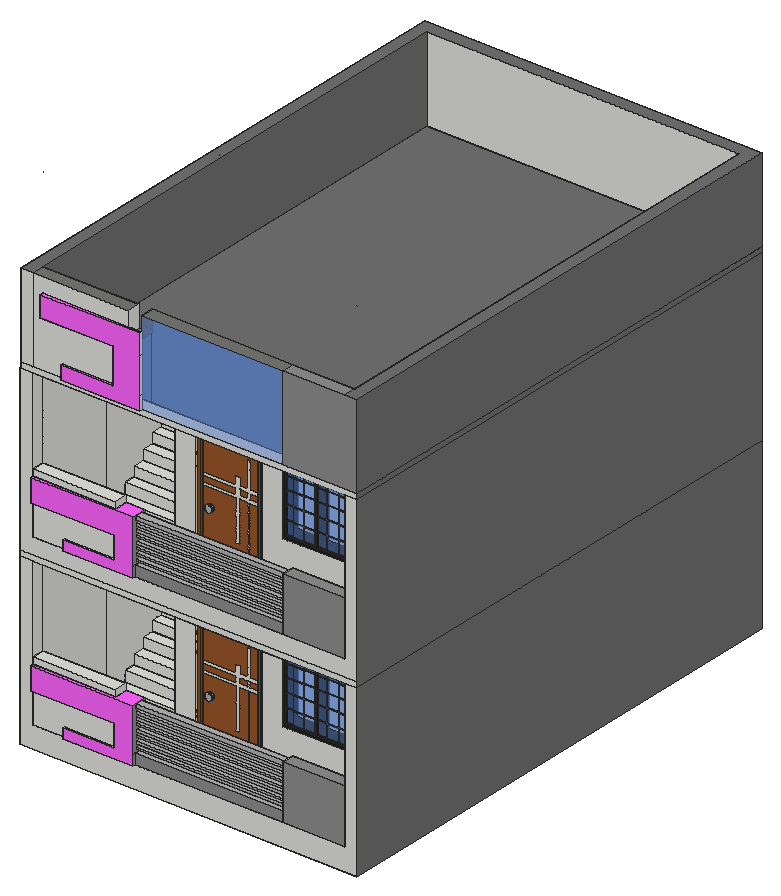
# SketchUp Ruby script. Lengths in inches.
U = 1.inch
M = Sketchup.active_model
def pt(a) = Geom::Point3d.new(a.map { |v| v * U })
def face(e, loops, mat)
  f = e.add_face(loops[0].map { |a| pt(a) })
  loops[1..].each { |l| e.add_face(l.map { |a| pt(a) }).erase! }
  f.material = f.back_material = mat if mat
  f
end
# faces: each face lists its corners as indices into pts; further lists are holes
def faces(e, pts, list, mat = nil) = list.each { |f| face(e, (f[0].is_a?(Array) ? f : [f]).map { |l| l.map { |i| pts[i] } }, mat) }
# xy, xz, yz: faces in a plane at the given z, y or x. An outline is a flat list of corners, or four numbers for a rectangle; further outlines are holes
def ring(l) = l.size == 4 ? [[l[0], l[1]], [l[2], l[1]], [l[2], l[3]], [l[0], l[3]]] : l.each_slice(2).to_a
def flat(e, list, mat, &to3) = list.each { |f| face(e, (f[0].is_a?(Array) ? f : [f]).map { |l| ring(l).map { |u, v| to3.(u, v) } }, mat) }
def xy(e, z, list, mat = nil) = flat(e, list, mat) { |x, y| [x, y, z] }
def xz(e, y, list, mat = nil) = flat(e, list, mat) { |x, z| [x, y, z] }
def yz(e, x, list, mat = nil) = flat(e, list, mat) { |y, z| [x, y, z] }
def lines(e, pts, list) = list.each { |a, b| e.add_line(pt(pts[a]), pt(pts[b])) }
# prism: a flat outline (further loops are holes) pulled along v
def prism(e, loops, v, mat = nil)
  f = face(e, loops, mat); d = Geom::Vector3d.new(v.map { |x| x * U })
  f.pushpull(f.normal.samedirection?(d) ? d.length : -d.length)
end
def box(e, o, s, mat = nil) = prism(e, [[o, [o[0] + s[0], o[1], o[2]], [o[0] + s[0], o[1] + s[1], o[2]], [o[0], o[1] + s[1], o[2]]]], [0, 0, s[2]], mat)
def at(x, y, z, deg = 0) = Geom::Transformation.translation(pt([x, y, z])) * Geom::Transformation.rotation(ORIGIN, Z_AXIS, deg.degrees)
def axes(o, x, y, z) = Geom::Transformation.new([*x, 0, *y, 0, *z, 0, *pt(o).to_a, 1])
def part(name) = M.definitions.add(name)
# library, detail: a bought-in or finely detailed component or shape, given as its bounding box
def library(name, o, s) = part(name).tap { |d| box(d.entities, o, s) }
def detail(e, o, s) = box(e.add_group.entities, o, s)
def put(e, d, t, mat = nil) = e.add_instance(d, t).tap { |i| i.material = mat if mat }
def group(e, t, mat = nil) = e.add_group.tap { |g| g.transformation = t; g.material = mat if mat }.entities
root = M.entities
M.materials.add("[Aluminum]").color = [179, 179, 179]
M.materials.add("[Color C07]").color = [153, 76, 0]
M.materials.add("[Color K03]").color = [255, 101, 255]
M.materials.add("[Color M04]").color = [142, 142, 142]
M.materials.add("[Color M05]").color = [114, 114, 114]
M.materials.add("[Color M08]").color = [30, 30, 30]
M.materials.add("[Metal Seamed]").color = [118, 119, 115]
M.materials.add("[Translucent Glass Blue]").color = [100, 149, 237]
M.materials["[Translucent Glass Blue]"].alpha = 0.5
M.materials.add("[Wood Cherry Original]").color = [152, 86, 42]
c1 = part("Group\#1")
xy(c1.entities,0,[[0,0,48,2],[0,2,48,11]],"[Color C07]")
xy(c1.entities,3,[[3,2,45,11]])
xy(c1.entities,3,[[3,0,45,2]],"[Color C07]")
xy(c1.entities,81,[[3,2,45,11]])
xy(c1.entities,81,[[3,0,45,2]],"[Color C07]")
xy(c1.entities,84,[[0,0,48,2],[0,2,48,11]],"[Color C07]")
xz(c1.entities,0,[[8.6,33.24,9.28,33.33,9.92,33.6,10.46,34.01,10.88,34.56,11.14,35.1875,11.23,35.87,11.14,36.55,10.88,37.18,10.46,37.72,9.92,38.14,9.28,38.4,8.6,38.49,7.92,38.4,7.29,38.14,6.75,37.72,6.33,37.18,6.07,36.55,5.98,35.87,6.07,35.1875,6.33,34.56,6.75,34.01,7.29,33.6,7.92,33.33]],"[Aluminum]")
xz(c1.entities,0,[[[0,0,48,84],[3,3,45,81]]],"[Color C07]")
xz(c1.entities,2,[[[0,0,48,84],[3,3,45,81]],[[35.64,15.58,37.45,15.58,37.45,48.41,45,48.41,45,50.73,37.45,50.73,37.45,54.78,45,54.78,45,57.1,37.45,57.1,37.45,75.83,35.64,75.83,35.64,57.1,29.69,57.1,29.69,62.31,27.44,62.31,27.44,57.1,3,57.1,3,54.78,27.44,54.78,27.44,50.73,3,50.73,3,48.41,27.44,48.41,27.44,19.68,29.69,19.68,29.69,48.41,35.64,48.41],[29.69,50.73,35.64,54.78]]])
xz(c1.entities,2,[[[3,3,45,3,45,48.41,37.45,48.41,37.45,15.58,35.64,15.58,35.64,48.41,29.69,48.41,29.69,19.68,27.44,19.68,27.44,48.41,3,48.41],[8.6,33.24,7.92,33.33,7.29,33.6,6.75,34.01,6.33,34.56,6.07,35.1875,5.98,35.87,6.07,36.55,6.33,37.18,6.75,37.72,7.29,38.14,7.92,38.4,8.6,38.49,9.28,38.4,9.92,38.14,10.46,37.72,10.88,37.18,11.14,36.55,11.23,35.87,11.14,35.1875,10.88,34.56,10.46,34.01,9.92,33.6,9.28,33.33]],[8.6,33.24,7.92,33.33,7.29,33.6,6.75,34.01,6.33,34.56,6.07,35.1875,5.98,35.87,6.07,36.55,6.33,37.18,6.75,37.72,7.29,38.14,7.92,38.4,8.6,38.49,9.28,38.4,9.92,38.14,10.46,37.72,10.88,37.18,11.14,36.55,11.23,35.87,11.14,35.1875,10.88,34.56,10.46,34.01,9.92,33.6,9.28,33.33],[3,50.73,27.44,54.78],[29.69,50.73,35.64,54.78],[37.45,50.73,45,54.78],
  [3,57.1,27.44,57.1,27.44,62.31,29.69,62.31,29.69,57.1,35.64,57.1,35.64,75.83,37.45,75.83,37.45,57.1,45,57.1,45,81,3,81]],"[Wood Cherry Original]")
xz(c1.entities,11,[[[0,0,48,84],[3,3,45,81]]])
yz(c1.entities,0,[[0,0,2,84],[2,0,11,84]],"[Color C07]")
yz(c1.entities,3,[[2,3,11,81]])
yz(c1.entities,3,[[0,3,2,81]],"[Color C07]")
yz(c1.entities,45,[[2,3,11,81]])
yz(c1.entities,45,[[0,3,2,81]],"[Color C07]")
yz(c1.entities,48,[[0,0,2,84],[2,0,11,84]],"[Color C07]")
p = [[7.92,2,33.33],[8.6,2,33.24],[8.6,0,33.24],[7.92,0,33.33],[9.28,2,33.33],[9.28,0,33.33],
  [7.29,2,33.6],[7.29,0,33.6],[9.92,2,33.6],[9.92,0,33.6],[6.75,2,34.01],[6.75,0,34.01],
  [10.46,2,34.01],[10.46,0,34.01],[6.33,2,34.56],[6.33,0,34.56],[10.88,2,34.56],[10.88,0,34.56],
  [6.07,2,35.1875],[6.07,0,35.1875],[11.14,2,35.1875],[11.14,0,35.1875],[5.98,2,35.87],[5.98,0,35.87],
  [11.23,2,35.87],[11.23,0,35.87],[6.07,2,36.55],[6.07,0,36.55],[11.14,2,36.55],[11.14,0,36.55],
  [6.33,2,37.18],[6.33,0,37.18],[10.88,2,37.18],[10.88,0,37.18],[6.75,2,37.72],[6.75,0,37.72],
  [10.46,2,37.72],[10.46,0,37.72],[7.29,2,38.14],[7.29,0,38.14],[9.92,2,38.14],[9.92,0,38.14],
  [7.92,2,38.4],[7.92,0,38.4],[9.28,2,38.4],[9.28,0,38.4],[8.6,2,38.49],[8.6,0,38.49]]
faces(c1.entities,p,[[0,1,2,3],[1,4,5,2],[6,0,3,7],[4,8,9,5],[10,6,7,11],[8,12,13,9],[14,10,11,15],[12,16,17,13],
  [18,14,15,19],[16,20,21,17],[22,18,19,23],[20,24,25,21],[26,22,23,27],[24,28,29,25],[30,26,27,31],[28,32,33,29],
  [34,30,31,35],[32,36,37,33],[38,34,35,39],[36,40,41,37],[42,38,39,43],[40,44,45,41],[46,42,43,47],[44,46,47,45]],"[Aluminum]")
c2 = part("Group\#2")
xy(c2.entities,0,[[0,0,48,11]])
xy(c2.entities,2,[[2,0,5.91,2],[5.91,0,6.35,2],[6.35,0,13.47,2],[13.47,0,13.91,2],[13.91,0,23.03,2],
  [24.15,0,29.6,2],[29.6,0,30.03,2],[30.03,0,38.16,2],[38.16,0,38.6,2],[38.6,0,46,2],
  [2,2,5.91,11],[5.91,2,6.35,11],[6.35,2,13.47,11],[13.47,2,13.91,11],[13.91,2,23.03,11],
  [24.15,2,29.6,11],[29.6,2,30.03,11],[30.03,2,38.16,11],[38.16,2,38.6,11],[38.6,2,46,11]])
xy(c2.entities,46,[[2,0,5.91,2],[5.91,0,6.35,2],[6.35,0,13.47,2],[13.47,0,13.91,2],[13.91,0,23.03,2],
  [24.15,0,29.6,2],[29.6,0,30.03,2],[30.03,0,38.16,2],[38.16,0,38.6,2],[38.6,0,46,2],
  [2,2,5.91,11],[5.91,2,6.35,11],[6.35,2,13.47,11],[13.47,2,13.91,11],[13.91,2,23.03,11],
  [24.15,2,29.6,11],[29.6,2,30.03,11],[30.03,2,38.16,11],[38.16,2,38.6,11],[38.6,2,46,11]])
xy(c2.entities,48,[[0,0,48,11]])
xz(c2.entities,0,[[[0,0,48,48],[24.15,2,46,46],[2,2,23.03,46]]],"[Color M08]")
xz(c2.entities,2,[[2,2,5.91,10.99],[[5.91,2,6.35,2,6.35,10.99,13.47,10.99,13.47,2,13.91,2,13.91,10.99,23.03,10.99,23.03,11.58,13.91,11.58,13.91,21.05,23.03,21.05,23.03,21.64,13.91,21.64,13.91,30.55,23.03,30.55,23.03,31.14,13.91,31.14,13.91,39.49,23.03,39.49,23.03,40.08,13.91,40.08,13.91,46,13.47,46,13.47,40.08,6.35,40.08,6.35,46,5.91,46,5.91,40.08,2,40.08,2,39.49,5.91,39.49,5.91,31.14,2,31.14,2,30.55,5.91,30.55,5.91,21.64,2,21.64,2,21.05,5.91,21.05,5.91,11.58,2,11.58,2,10.99,5.91,10.99],[6.35,11.58,13.47,21.05],[6.35,21.64,13.47,30.55],[6.35,31.14,13.47,39.49]],[6.35,2,13.47,10.99],[13.91,2,23.03,10.99],[24.15,2,29.6,10.99],
  [[29.6,2,30.03,2,30.03,10.99,38.16,10.99,38.16,2,38.6,2,38.6,10.99,46,10.99,46,11.58,38.6,11.58,38.6,21.05,46,21.05,46,21.64,38.6,21.64,38.6,30.55,46,30.55,46,31.14,38.6,31.14,38.6,39.49,46,39.49,46,40.08,38.6,40.08,38.6,46,38.16,46,38.16,40.08,30.03,40.08,30.03,46,29.6,46,29.6,40.08,24.15,40.08,24.15,39.49,29.6,39.49,29.6,31.14,24.15,31.14,24.15,30.55,29.6,30.55,29.6,21.64,24.15,21.64,24.15,21.05,29.6,21.05,29.6,11.58,24.15,11.58,24.15,10.99,29.6,10.99],[30.03,11.58,38.16,21.05],[30.03,21.64,38.16,30.55],[30.03,31.14,38.16,39.49]],[30.03,2,38.16,10.99],[38.6,2,46,10.99],[2,11.58,5.91,21.05],[6.35,11.58,13.47,21.05],
  [13.91,11.58,23.03,21.05],[24.15,11.58,29.6,21.05],[30.03,11.58,38.16,21.05],[38.6,11.58,46,21.05],[2,21.64,5.91,30.55],
  [6.35,21.64,13.47,30.55],[13.91,21.64,23.03,30.55],[24.15,21.64,29.6,30.55],[30.03,21.64,38.16,30.55],[38.6,21.64,46,30.55],
  [2,31.14,5.91,39.49],[6.35,31.14,13.47,39.49],[13.91,31.14,23.03,39.49],[24.15,31.14,29.6,39.49],[30.03,31.14,38.16,39.49],
  [38.6,31.14,46,39.49],[2,40.08,5.91,46],[6.35,40.08,13.47,46],[13.91,40.08,23.03,46],[24.15,40.08,29.6,46],
  [30.03,40.08,38.16,46],[38.6,40.08,46,46]],"[Translucent Glass Blue]")
xz(c2.entities,11,[[[0,0,48,48],[2,2,46,46]],[23.03,2,24.15,46]])
xz(c2.entities,11,[[2,2,23.03,46],[24.15,2,46,46]],"[Translucent Glass Blue]")
yz(c2.entities,0,[[0,0,11,48]])
yz(c2.entities,2,[[0,2,2,10.99],[2,2,11,46],[0,10.99,2,11.58],[0,11.58,2,21.05],[0,21.05,2,21.64],
  [0,21.64,2,30.55],[0,30.55,2,31.14],[0,31.14,2,39.49],[0,39.49,2,40.08],[0,40.08,2,46]])
yz(c2.entities,23.03,[[0,2,2,21.05],[2,2,11,46],[0,21.05,2,21.64],[0,21.64,2,30.55],[0,30.55,2,31.14],
  [0,31.14,2,46]])
yz(c2.entities,24.15,[[0,2,2,10.99],[2,2,11,46],[0,10.99,2,11.58],[0,11.58,2,21.05],[0,21.05,2,21.64],
  [0,21.64,2,30.55],[0,30.55,2,31.14],[0,31.14,2,46]])
yz(c2.entities,46,[[0,2,2,10.99],[2,2,11,46],[0,10.99,2,11.58],[0,11.58,2,21.05],[0,21.05,2,21.64],
  [0,21.64,2,30.55],[0,30.55,2,31.14],[0,31.14,2,39.49],[0,39.49,2,40.08],[0,40.08,2,46]])
yz(c2.entities,48,[[0,0,11,48]])
c3 = part("Group\#4")
box(c3.entities,[0,0,0],[24,12,6])
c4 = part("Group\#5")
put(c4.entities,c3,at(0,192,96))
put(c4.entities,c3,at(0,168,84))
put(c4.entities,c3,at(0,180,90))
put(c4.entities,c3,at(0,108,54))
put(c4.entities,c3,at(0,120,60))
put(c4.entities,c3,at(0,12,6))
put(c4.entities,c3,at(0,0,0))
put(c4.entities,c3,at(0,132,66))
put(c4.entities,c3,at(0,156,78))
put(c4.entities,c3,at(0,144,72))
put(c4.entities,c3,at(0,60,30))
put(c4.entities,c3,at(0,84,42))
put(c4.entities,c3,at(0,36,18))
put(c4.entities,c3,at(0,48,24))
put(c4.entities,c3,at(0,96,48))
put(c4.entities,c3,at(0,72,36))
g1 = group(c4.entities,at(0,24,12))
box(g1,[0,0,0],[24,12,6])
xy(root,0,[[[0,2,240,362],[9,11,231,353]],[[9,11,231,11,231,59,126,59,126,68,231,68,231,353,9,353],[64.18,59,79.6875,68]],[64.18,59,79.6875,68],[126,59,141.5625,68],[141.5625,59,231,68]])
xy(root,15.8125,[[32.07,0,68.09,2],[68.09,0,81.64,2],[9,2,68.09,11],[68.09,2,81.64,11],[81.64,2,186.77,11],
  [186.77,2,231,11]])
xy(root,22.36,[[32.07,0,68.09,2]])
xy(root,23.0625,[[68.09,2,81.64,11],[68.09,11,81.64,11.3125]])
xy(root,23.0625,[[81.64,2,186.77,11]],"[Aluminum]")
xy(root,25.13,[[81.64,3.26,187.95,8.32]])
xy(root,26.75,[[81.64,3.26,187.95,8.32]],"[Aluminum]")
xy(root,28.69,[[81.64,3.26,186.77,8.32]])
xy(root,30.32,[[81.64,3.26,186.77,8.32]],"[Aluminum]")
xy(root,32.57,[[81.64,3.26,191.14,8.32]])
xy(root,34.19,[[81.64,3.26,191.14,8.32]],"[Aluminum]")
xy(root,36,[[141.5625,59,189.5625,68]])
xy(root,36.19,[[81.64,3.26,188.26,8.32]])
xy(root,37.82,[[81.64,3.26,188.26,8.32]],"[Aluminum]")
xy(root,38.16,[[9,0,68.09,2]])
xy(root,40.25,[[81.64,3.26,186.77,8.32]])
xy(root,41.88,[[81.64,3.26,186.77,8.32]],"[Aluminum]")
xy(root,43.73,[[81.64,3.01,189.45,8.2]])
xy(root,45.73,[[81.64,3.01,189.45,8.2]],"[Aluminum]")
xy(root,47.73,[[81.64,3.01,195.01,8.2]])
xy(root,49.73,[[81.64,3.01,195.01,8.2]],"[Aluminum]")
xy(root,51.375,[[81.64,2.84,186.89,7.97]])
xy(root,54.375,[[186.77,2.84,186.89,7.97]])
xy(root,54.375,[[81.64,2.84,186.77,7.97]],"[Aluminum]")
xy(root,54.375,[[9,0,81.64,0,81.64,11.3125,68.09,11.3125,68.09,2,9,2]],"[Color K03]")
xy(root,54.375,[[186.77,2,231,2,231,11,186.77,11,186.77,7.97,186.89,7.97,186.89,2.84,186.77,2.84]],"[Color M04]")
xy(root,58.9375,[[9,2,68.09,11]])
xy(root,84,[[79.6875,59,126,68],[141.5625,59,189.5625,68]])
xy(root,120,[[0,2,9,2,9,353,231,353,231,2,239.875,2,239.875,362,0,362],[9,2,231,11],[239.875,2,240,362],[9,11,231,11,231,59,64.18,59,64.18,68,231,68,231,353,9,353],[64.18,59,79.6875,68],
  [79.6875,59,126,68],[126,59,141.5625,68],[141.5625,59,231,68],[0,362,239.875,362.125]])
xy(root,124,[[0,2,239.875,362.125]])
xy(root,135.8125,[[32.07,0,68.09,2],[68.09,0,81.64,2],[9,2,68.09,11],[68.09,2,81.64,11],[81.64,2,186.77,11],
  [186.77,2,231,11]])
xy(root,142.36,[[32.07,0,68.09,2]])
xy(root,143.0625,[[68.09,2,81.64,11],[68.09,11,81.64,11.3125]])
xy(root,143.0625,[[81.64,2,186.77,11]],"[Aluminum]")
xy(root,145.13,[[81.64,3.26,187.95,8.32]])
xy(root,146.75,[[81.64,3.26,187.95,8.32]],"[Aluminum]")
xy(root,148.69,[[81.64,3.26,186.77,8.32]])
xy(root,150.32,[[81.64,3.26,186.77,8.32]],"[Aluminum]")
xy(root,152.57,[[81.64,3.26,191.14,8.32]])
xy(root,154.19,[[81.64,3.26,191.14,8.32]],"[Aluminum]")
xy(root,156,[[141.5625,59,189.5625,68]])
xy(root,156.19,[[81.64,3.26,188.26,8.32]])
xy(root,157.82,[[81.64,3.26,188.26,8.32]],"[Aluminum]")
xy(root,158.16,[[9,0,68.09,2]])
xy(root,160.25,[[81.64,3.26,186.77,8.32]])
xy(root,161.88,[[81.64,3.26,186.77,8.32]],"[Aluminum]")
xy(root,163.73,[[81.64,3.01,189.45,8.2]])
xy(root,165.73,[[81.64,3.01,189.45,8.2]],"[Aluminum]")
xy(root,167.73,[[81.64,3.01,195.01,8.2]])
xy(root,169.73,[[81.64,3.01,195.01,8.2]],"[Aluminum]")
xy(root,171.375,[[81.64,2.84,186.89,7.97]])
xy(root,174.375,[[186.77,2.84,186.89,7.97]])
xy(root,174.375,[[81.64,2.84,186.77,7.97]],"[Aluminum]")
xy(root,174.375,[[9,0,81.64,0,81.64,11.3125,68.09,11.3125,68.09,2,9,2]],"[Color K03]")
xy(root,174.375,[[186.77,2,231,2,231,11,186.77,11,186.77,7.97,186.89,7.97,186.89,2.84,186.77,2.84]],"[Color M04]")
xy(root,178.9375,[[9,2,68.09,11]])
xy(root,204,[[79.6875,59,126,68],[141.5625,59,189.5625,68]])
xy(root,240,[[0,2,0.125,362],[0.125,2,0.125,362,240,362,240,2,231,2,231,353,9,353,9,2],[9,2,9,353,231,353,231,68,64.18,68,64.18,59,231,59,231,2],[64.18,59,231,68]])
xy(root,244,[[30.36,0,68.09,2],[68.09,0,86.45,2],[[0.125,2,240,362],[9.125,11,231,353]]])
xy(root,244,[[9.125,11,231,353]],"[Color M05]")
xy(root,253.54,[[67.89,0,68.09,2]])
xy(root,253.54,[[30.36,0,67.89,2]],"[Color K03]")
xy(root,278.9,[[15.84,0,67.89,2]])
xy(root,288.75,[[77.34,2,86.45,11]],"[Color M04]")
xy(root,293.53,[[15.84,0,86.45,2]],"[Color K03]")
xy(root,304,[[186.77,2,231,11]],"[Color M04]")
xy(root,304,[[0.125,2,9.125,2,9.125,353,231,353,231,2,240,2,240,362,0.125,362]],"[Color M05]")
xy(root,304,[[9.125,2,77.34,11],[86.45,2,186.77,11]],"[Metal Seamed]")
xz(root,0,[[32.07,15.8125,81.64,15.8125,81.64,54.375,9,54.375,9,38.16,68.09,38.16,68.09,22.36,32.07,22.36],[32.07,135.8125,81.64,135.8125,81.64,174.375,9,174.375,9,158.16,68.09,158.16,68.09,142.36,32.07,142.36],[30.36,244,86.45,244,86.45,293.53,15.84,293.53,15.84,278.9,67.89,278.9,67.89,253.54,30.36,253.54]],"[Color K03]")
xz(root,2,[[0,0,240,0,240,120,231,120,231,15.8125,9,15.8125,9,120,0,120],[9,15.8125,32.07,15.8125,32.07,22.36,68.09,22.36,68.09,38.16,9,38.16],[68.09,15.8125,81.64,23.0625],[9,38.16,68.09,54.375],[9,54.375,68.09,58.9375],
  [0,120,239.875,124],[239.875,120,240,120,240,240,231,240,231,135.8125,9,135.8125,9,240,0,240,0,124,239.875,124],[9,135.8125,32.07,135.8125,32.07,142.36,68.09,142.36,68.09,158.16,9,158.16],[68.09,135.8125,81.64,143.0625],[9,158.16,68.09,174.375],
  [9,174.375,68.09,178.9375],[0.125,240,240,244],[0.125,244,9.125,304],[9.125,244,30.36,244,30.36,253.54,67.89,253.54,67.89,278.9,15.84,278.9,15.84,293.53,77.34,293.53,77.34,304,9.125,304],[67.89,253.54,68.09,278.9],
  [77.34,288.75,86.45,293.53]])
xz(root,2,[[81.64,15.8125,186.77,23.0625],[186.77,15.8125,231,54.375],[81.64,135.8125,186.77,143.0625],[186.77,135.8125,231,174.375],[186.77,244,240,304]],"[Color M04]")
xz(root,2,[[86.45,244,186.77,304]],"[Translucent Glass Blue]")
xz(root,2.84,[[81.64,51.375,186.89,54.375],[81.64,171.375,186.89,174.375]],"[Aluminum]")
xz(root,3.01,[[81.64,43.73,189.45,45.73],[81.64,47.73,195.01,49.73],[81.64,163.73,189.45,165.73],[81.64,167.73,195.01,169.73]],"[Aluminum]")
xz(root,3.26,[[81.64,25.13,187.95,26.75],[81.64,28.69,186.77,30.32],[81.64,32.57,191.14,34.19],[81.64,36.19,188.26,37.82],[81.64,40.25,186.77,41.88],
  [81.64,145.13,187.95,146.75],[81.64,148.69,186.77,150.32],[81.64,152.57,191.14,154.19],[81.64,156.19,188.26,157.82],[81.64,160.25,186.77,161.88]],"[Aluminum]")
xz(root,7.97,[[81.64,51.375,186.89,54.375],[81.64,171.375,186.89,174.375]],"[Aluminum]")
xz(root,8.2,[[81.64,43.73,189.45,45.73],[81.64,47.73,195.01,49.73],[81.64,163.73,189.45,165.73],[81.64,167.73,195.01,169.73]],"[Aluminum]")
xz(root,8.32,[[81.64,25.13,187.95,26.75],[81.64,28.69,186.77,30.32],[81.64,32.57,191.14,34.19],[81.64,36.19,188.26,37.82],[81.64,40.25,186.77,41.88],
  [81.64,145.13,187.95,146.75],[81.64,148.69,186.77,150.32],[81.64,152.57,191.14,154.19],[81.64,156.19,188.26,157.82],[81.64,160.25,186.77,161.88]],"[Aluminum]")
xz(root,11,[[9,0,231,15.8125],[9,15.8125,68.09,58.9375],[68.09,15.8125,81.64,23.0625],[81.64,15.8125,186.77,23.0625],[186.77,15.8125,231,54.375],
  [9,120,231,135.8125],[9,135.8125,68.09,178.9375],[68.09,135.8125,81.64,143.0625],[81.64,135.8125,186.77,143.0625],[186.77,135.8125,231,174.375]])
xz(root,11,[[9.125,244,9.125,304,77.34,304,77.34,288.75,68.09,288.75,68.09,244],[186.77,244,231,304]],"[Color M05]")
xz(root,11,[[68.09,244,86.45,288.75],[86.45,244,186.77,304]],"[Translucent Glass Blue]")
xz(root,11.3125,[[68.09,23.0625,81.64,54.375],[68.09,143.0625,81.64,174.375]])
xz(root,59,[[[64.18,0,79.6875,0,79.6875,84,126,84,126,0,231,0,231,120,64.18,120],[141.5625,36,189.5625,84]],[[64.18,120,79.6875,120,79.6875,204,126,204,126,120,231,120,231,240,64.18,240],[141.5625,156,189.5625,204]]])
xz(root,68,[[[64.18,0,64.18,120,231,120,231,0,126,0,126,84,79.6875,84,79.6875,0],[141.5625,36,189.5625,84]],[[64.18,120,64.18,240,231,240,231,120,126,120,126,204,79.6875,204,79.6875,120],[141.5625,156,189.5625,204]]])
xz(root,353,[[9,0,231,120],[9,120,231,240],[9.125,244,231,304]])
xz(root,362,[[0,0,240,120],[0,120,240,240],[0.125,240,240,244],[0.125,244,240,304]])
xz(root,362.125,[[0,120,239.875,124]])
yz(root,0,[[362,120,362.125,124]])
yz(root,0,[[2,0,362,120],[2,120,362,124],[2,124,362,240]],"[Color M05]")
yz(root,0.125,[[2,240,362,244],[2,244,362,304]],"[Color M05]")
yz(root,9,[[11,0,68,120],[68,0,353,120],[2,15.8125,11,58.9375],[0,38.16,2,54.375],[2,58.9375,11,120],
  [11,120,68,240],[68,120,353,240],[2,135.8125,11,178.9375],[0,158.16,2,174.375],[2,178.9375,11,240]])
yz(root,9.125,[[11,244,353,304]],"[Color M05]")
yz(root,15.84,[[0,278.9,2,293.53]],"[Color K03]")
yz(root,30.36,[[0,244,2,253.54]],"[Color K03]")
yz(root,32.07,[[0,15.8125,2,22.36],[0,135.8125,2,142.36]])
yz(root,64.18,[[59,0,68,120],[59,120,68,240]])
yz(root,67.89,[[0,253.54,2,278.9]],"[Color K03]")
yz(root,68.09,[[0,22.36,2,38.16],[2,23.0625,11,38.16],[11,23.0625,11.3125,38.16],[2,38.16,11,54.375],[11,38.16,11.3125,54.375],
  [2,54.375,11,58.9375],[0,142.36,2,158.16],[2,143.0625,11,158.16],[11,143.0625,11.3125,158.16],[2,158.16,11,174.375],
  [11,158.16,11.3125,174.375],[2,174.375,11,178.9375]])
yz(root,77.34,[[2,288.75,11,304]])
yz(root,79.6875,[[59,0,68,84],[59,120,68,204]])
yz(root,81.64,[[2,15.8125,11,23.0625],[2.84,51.375,7.97,54.375],[2,135.8125,11,143.0625],[2.84,171.375,7.97,174.375]])
yz(root,81.64,[[0,15.8125,2,23.0625],[[0,23.0625,11.3125,23.0625,11.3125,54.375,7.97,54.375,7.97,51.375,2.84,51.375,2.84,54.375,0,54.375],[3.01,43.73,8.2,45.73],[3.01,47.73,8.2,49.73],[3.26,25.13,8.32,26.75],[3.26,28.69,8.32,30.32],[3.26,32.57,8.32,34.19],[3.26,36.19,8.32,37.82],[3.26,40.25,8.32,41.88]],[0,135.8125,2,143.0625],[[0,143.0625,11.3125,143.0625,11.3125,174.375,7.97,174.375,7.97,171.375,2.84,171.375,2.84,174.375,0,174.375],[3.01,163.73,8.2,165.73],[3.01,167.73,8.2,169.73],[3.26,145.13,8.32,146.75],[3.26,148.69,8.32,150.32],[3.26,152.57,8.32,154.19],[3.26,156.19,8.32,157.82],[3.26,160.25,8.32,161.88]]],"[Color M04]")
yz(root,86.45,[[0,244,2,253.54],[0,253.54,2,278.9],[0,278.9,2,293.53]])
yz(root,86.45,[[2,288.75,11,304]],"[Metal Seamed]")
yz(root,126,[[59,0,68,84],[59,120,68,204]])
yz(root,141.5625,[[59,36,68,84],[59,156,68,204]])
yz(root,186.77,[[2,15.8125,11,23.0625],[2,135.8125,11,143.0625]])
yz(root,186.77,[[[2,23.0625,11,54.375],[3.26,28.69,8.32,30.32],[3.26,40.25,8.32,41.88]],[[2,143.0625,11,174.375],[3.26,148.69,8.32,150.32],[3.26,160.25,8.32,161.88]]],"[Color M04]")
yz(root,186.89,[[2.84,51.375,7.97,54.375],[2.84,171.375,7.97,174.375]])
yz(root,187.95,[[3.26,25.13,8.32,26.75],[3.26,145.13,8.32,146.75]])
yz(root,188.26,[[3.26,36.19,8.32,37.82],[3.26,156.19,8.32,157.82]])
yz(root,189.45,[[3.01,43.73,8.2,45.73],[3.01,163.73,8.2,165.73]])
yz(root,189.5625,[[59,36,68,84],[59,156,68,204]])
yz(root,191.14,[[3.26,32.57,8.32,34.19],[3.26,152.57,8.32,154.19]])
yz(root,195.01,[[3.01,47.73,8.2,49.73],[3.01,167.73,8.2,169.73]])
yz(root,231,[[11,0,59,120],[59,0,68,120],[68,0,353,120],[2,15.8125,11,54.375],[2,54.375,11,120],
  [11,120,59,240],[59,120,68,240],[68,120,353,240],[2,135.8125,11,174.375],[2,174.375,11,240],
  [11,244,353,304]])
yz(root,239.875,[[2,120,362.125,124]])
yz(root,240,[[2,0,362,120],[2,120,362,240],[2,240,362,244],[2,244,362,304]],"[Color M05]")
p = [[338.11,-308.57,-0.03],[337.68,-308.57,-0.03],[73.62,87.23,365],[73.62,87.23,364],[240,2,364],[239.56,2,364],
  [68.09,2,278.9],[86.45,2,278.9],[9.125,11,365.125],[9.125,11,364]]
lines(root,p,[[0,1],[2,3],[4,5],[6,7],[8,9]])
put(root,c1,axes([79.6875,59.45,120],[0.97449,0,0],[0,0.9595,0],[0,0,1]))
put(root,c2,at(141.5625,59,156),"[Color M08]")
put(root,c4,axes([9,75.92,120],[1.9,0,0],[0,0.6666,0],[0,0,1.2]))
put(root,c4,axes([9,75.92,0],[1.9,0,0],[0,0.6666,0],[0,0,1.2]))
put(root,c1,axes([79.6875,59.45,0],[0.97449,0,0],[0,0.9595,0],[0,0,1]))
put(root,c2,at(141.5625,59,36),"[Color M08]")
